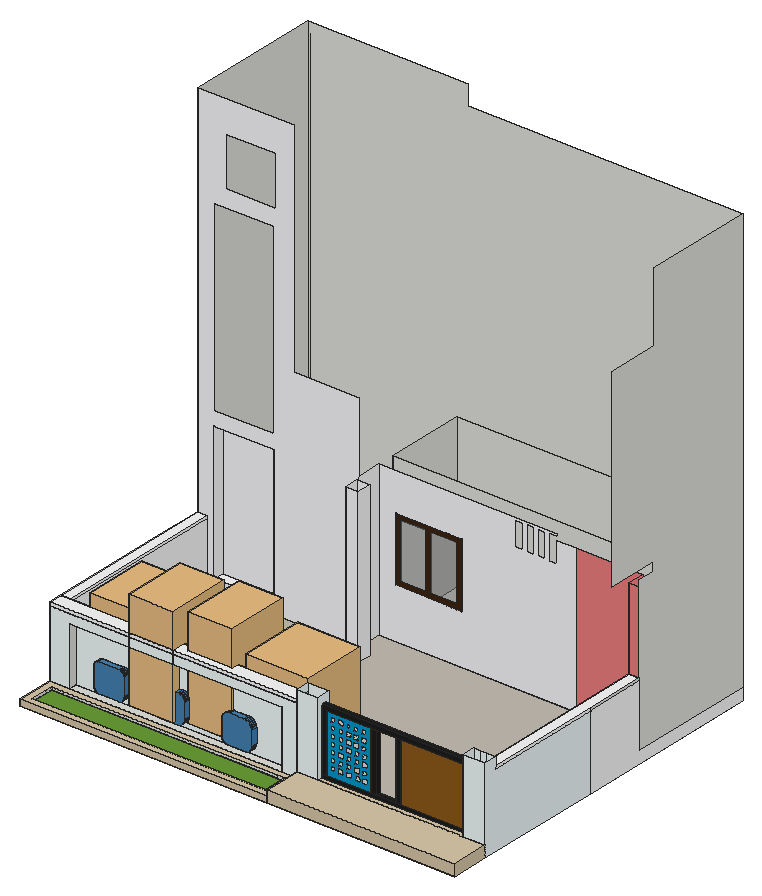
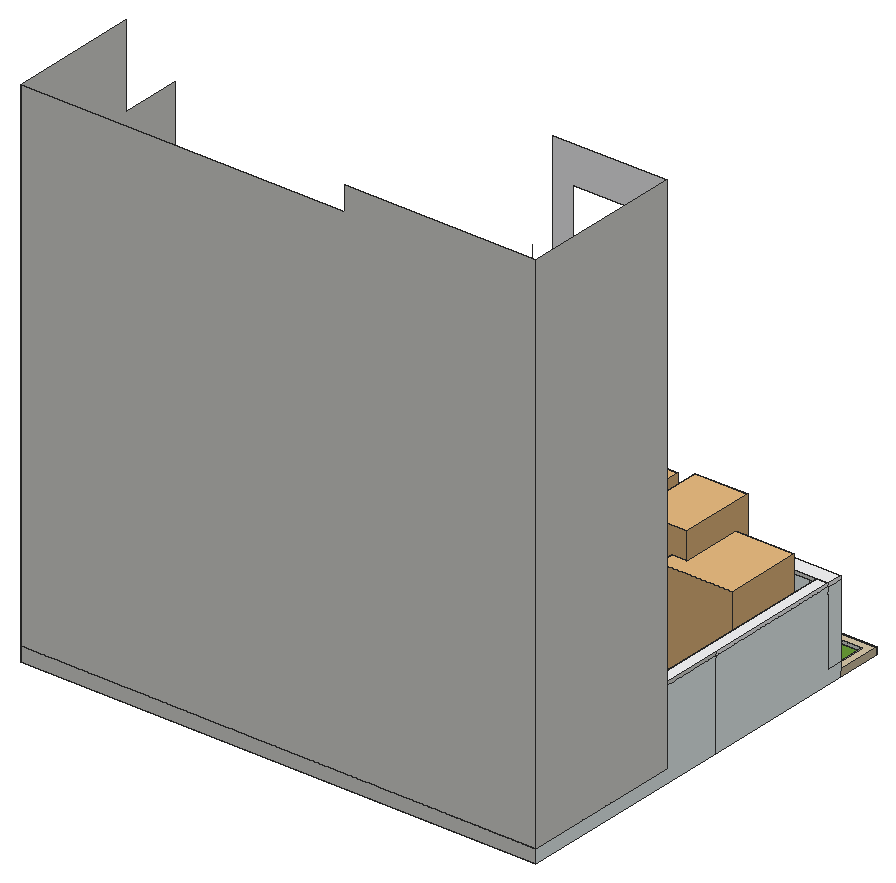
# SketchUp Ruby script. Lengths in inches.
U = 1.inch
M = Sketchup.active_model
def pt(a) = Geom::Point3d.new(a.map { |v| v * U })
def face(e, loops, mat)
  f = e.add_face(loops[0].map { |a| pt(a) })
  loops[1..].each { |l| e.add_face(l.map { |a| pt(a) }).erase! }
  f.material = f.back_material = mat if mat
  f
end
# faces: each face lists its corners as indices into pts; further lists are holes
def faces(e, pts, list, mat = nil) = list.each { |f| face(e, (f[0].is_a?(Array) ? f : [f]).map { |l| l.map { |i| pts[i] } }, mat) }
# xy, xz, yz: faces in a plane at the given z, y or x. An outline is a flat list of corners, or four numbers for a rectangle; further outlines are holes
def ring(l) = l.size == 4 ? [[l[0], l[1]], [l[2], l[1]], [l[2], l[3]], [l[0], l[3]]] : l.each_slice(2).to_a
def flat(e, list, mat, &to3) = list.each { |f| face(e, (f[0].is_a?(Array) ? f : [f]).map { |l| ring(l).map { |u, v| to3.(u, v) } }, mat) }
def xy(e, z, list, mat = nil) = flat(e, list, mat) { |x, y| [x, y, z] }
def xz(e, y, list, mat = nil) = flat(e, list, mat) { |x, z| [x, y, z] }
def yz(e, x, list, mat = nil) = flat(e, list, mat) { |y, z| [x, y, z] }
def lines(e, pts, list) = list.each { |a, b| e.add_line(pt(pts[a]), pt(pts[b])) }
# prism: a flat outline (further loops are holes) pulled along v
def prism(e, loops, v, mat = nil)
  f = face(e, loops, mat); d = Geom::Vector3d.new(v.map { |x| x * U })
  f.pushpull(f.normal.samedirection?(d) ? d.length : -d.length)
end
def box(e, o, s, mat = nil) = prism(e, [[o, [o[0] + s[0], o[1], o[2]], [o[0] + s[0], o[1] + s[1], o[2]], [o[0], o[1] + s[1], o[2]]]], [0, 0, s[2]], mat)
def at(x, y, z, deg = 0) = Geom::Transformation.translation(pt([x, y, z])) * Geom::Transformation.rotation(ORIGIN, Z_AXIS, deg.degrees)
def axes(o, x, y, z) = Geom::Transformation.new([*x, 0, *y, 0, *z, 0, *pt(o).to_a, 1])
def part(name) = M.definitions.add(name)
# library, detail: a bought-in or finely detailed component or shape, given as its bounding box
def library(name, o, s) = part(name).tap { |d| box(d.entities, o, s) }
def detail(e, o, s) = box(e.add_group.entities, o, s)
def put(e, d, t, mat = nil) = e.add_instance(d, t).tap { |i| i.material = mat if mat }
def group(e, t, mat = nil) = e.add_group.tap { |g| g.transformation = t; g.material = mat if mat }.entities
root = M.entities
M.materials.add("[0013_LightCoral]").color = [255, 136, 136]
M.materials.add("[0013_LightCoral]1").color = [240, 128, 128]
M.materials.add("[0097_DeepSkyBlue]").color = [0, 152, 204]
M.materials.add("[0100_SteelBlue]").color = [70, 130, 180]
M.materials.add("[Blinds Vertical Pattern]").color = [250, 250, 252]
M.materials.add("[Blinds Weave]").color = [141, 91, 25]
M.materials.add("[Color M08]").color = [30, 30, 30]
M.materials.add("[Field Rectangle Tile]").color = [196, 189, 179]
M.materials.add("[Field Square Tile]").color = [217, 201, 169]
M.materials.add("[Grass Dark Green]").color = [106, 157, 55]
M.materials.add("[Translucent Glass Gray]").color = [128, 128, 128]
M.materials["[Translucent Glass Gray]"].alpha = 0.5
M.materials.add("[White Subway Tile]").color = [243, 252, 253]
M.materials.add("[Wood Cherry Original]").color = [66, 37, 18]
c1 = library("chau cay",[-24.34,-109.24,0],[56.46,62.58,79.69])
c2 = library("Flora+17",[-57.52,158.6,-38.64],[66.99,62.88,77.28])
xy(root,0,[[[5.9375,0,199.85,29.3125],[11.12,5.18,194.66,24.13]],[11.12,5.18,194.66,24.13],[5.9375,29.3125,5.9375,132.68,347.47,132.68,347.47,29.3125,187.7,29.3125,187.7,35.625,21.2,35.625,21.2,29.3125],[21.2,29.3125,187.7,35.625],[5.9375,132.68,347.47,281.71]])
xy(root,0,[[199.85,0,347.47,29.3125]],"[Field Square Tile]")
xy(root,2.5,[[11.12,5.18,194.66,24.13]],"[Grass Dark Green]")
xy(root,4.6875,[[21.2,29.3125,187.7,35.625]])
xy(root,4.6875,[[[5.9375,0,199.85,29.3125],[11.12,5.18,194.66,24.13]]],"[Field Square Tile]")
xy(root,7.5625,[[43.19,31.25,57.63,35.625],[92.19,31.25,104.38,35.625],[143.86,31.25,157.93,35.625]],"[0100_SteelBlue]")
xy(root,9,[[216.33,32.96,330.16,36.41],[216.33,36.41,330.16,39.87],[133.75,159.42,143.75,170.29],[5.9375,173.82,5.9375,281.71,347.47,281.71,347.47,180.38,339.34,180.38,339.34,194.19,308.22,194.19,308.22,207.2,339.34,207.2,339.34,270.27,17.38,270.27,17.38,173.82],[17.38,173.82,17.38,270.27,132.29,270.27,132.29,207.2,308.22,207.2,308.22,194.19,132.29,194.19,132.29,173.82],
  [132.29,207.2,339.34,270.27]])
xy(root,9,[[[13.63,39.87,339.34,39.87,339.34,194.19,132.29,194.19,132.29,173.82,13.63,173.82],[133.75,159.42,143.75,170.29]]],"[Field Rectangle Tile]")
xy(root,9,[[199.85,0,347.47,29.3125],[216.33,29.3125,330.16,32.96]],"[Field Square Tile]")
xy(root,11.5,[[216.33,32.96,219.96,36.41],[219.96,32.96,255,36.41],[255,32.96,259.13,36.41],[274.16,32.96,278.35,36.41],[278.35,32.96,326.78,36.41],
  [326.78,32.96,330.16,36.41]])
xy(root,11.5,[[259.13,32.96,274.16,36.41]],"[Color M08]")
xy(root,17.61,[[19.23,173.82,65.86,182.32]],"[Blinds Vertical Pattern]")
xy(root,30.1875,[[42.77,31.25,59.07,35.625],[91.14,31.25,105.43,35.625],[145.77,31.25,156.82,35.625]],"[0100_SteelBlue]")
xy(root,50.25,[[21.2,29.3125,187.7,35.625]])
xy(root,57.36,[[255,32.96,259.13,36.41],[274.16,32.96,278.35,36.41]])
xy(root,57.36,[[259.13,32.96,274.16,36.41]],"[Color M08]")
xy(root,57.5625,[[5.9375,29.3125,199.85,39.87]])
xy(root,58.0625,[[5.9375,39.87,13.63,173.82],[339.34,39.87,347.47,180.38]])
xy(root,60.25,[[5.9375,29.3125,199.85,39.87],[5.9375,39.87,13.63,173.82]],"[Blinds Vertical Pattern]")
xy(root,60.3125,[[339.34,39.87,347.47,180.38]],"[Blinds Vertical Pattern]")
xy(root,60.88,[[216.33,32.96,326.78,36.41],[326.78,32.96,330.16,36.41]],"[Color M08]")
xz(root,0,[[5.9375,0,199.85,4.6875],[199.85,0,347.47,9]],"[Field Square Tile]")
xz(root,5.18,[[11.12,0,194.66,2.5],[11.12,2.5,194.66,4.6875]])
xz(root,24.13,[[11.12,0,21.2,2.5],[21.2,0,187.7,2.5],[187.7,0,194.66,2.5],[11.12,2.5,21.2,4.6875],[21.2,2.5,187.7,4.6875],
  [187.7,2.5,194.66,4.6875]])
xz(root,29.3125,[[5.9375,0,21.2,4.6875],[21.2,0,187.7,4.6875],[187.7,0,199.85,4.6875],[199.85,0,216.33,9],[216.33,0,330.16,9],
  [330.16,0,347.47,9]])
xz(root,29.3125,[[5.9375,57.5625,199.85,60.25]],"[Blinds Vertical Pattern]")
xz(root,29.3125,[[5.9375,4.6875,21.2,4.6875,21.2,50.25,187.7,50.25,187.7,4.6875,199.85,4.6875,199.85,57.5625,5.9375,57.5625],[199.85,9,216.33,66.6875],[330.16,9,347.47,66.6875]],"[White Subway Tile]")
xz(root,31.25,[[43.19,7.5625,57.63,7.5625,58.31,7.61,58.97,7.74,59.61,7.96,60.21,8.25,60.77,8.63,61.28,9.07,61.72,9.58,62.1,10.14,62.4,10.75,62.61,11.39,62.75,12.05,62.79,12.72,62.79,26.47,62.76,26.96,62.66,27.43,62.51,27.89,62.29,28.33,62.02,28.73,61.7,29.1,61.34,29.42,60.93,29.69,60.5,29.91,60.04,30.0625,59.56,30.16,59.07,30.1875,42.77,30.1875,42.26,30.15,41.75,30.05,41.27,29.89,40.81,29.66,40.38,29.38,40,29.04,39.66,28.66,39.375,28.23,39.15,27.77,38.99,27.29,38.89,26.78,38.85,26.27,38.85,11.91,38.89,11.34,39,10.78,39.18,10.24,39.43,9.73,39.75,9.26,40.125,8.84,40.55,8.46,41.02,8.14,41.53,7.89,42.07,7.71,42.63,7.6],[92.19,7.5625,104.38,7.5625,105.17,7.61,105.94,7.77,106.69,8.02,107.4,8.37,108.05,8.81,108.65,9.33,109.17,9.92,109.61,10.58,109.96,11.29,110.21,12.03,110.36,12.81,110.41,13.59,110.41,25.21,110.37,25.86,110.24,26.5,110.04,27.11,109.75,27.7,109.39,28.24,108.96,28.73,108.47,29.16,107.92,29.52,107.34,29.81,106.72,30.02,106.08,30.15,105.43,30.1875,91.14,30.1875,90.53,30.15,89.93,30.03,89.36,29.83,88.81,29.5625,88.3,29.22,87.84,28.82,87.44,28.36,87.1,27.86,86.83,27.31,86.64,26.73,86.52,26.13,86.48,25.52,86.48,13.28,86.53,12.53,86.67,11.8,86.91,11.09,87.24,10.42,87.66,9.8,88.15,9.24,88.71,8.74,89.33,8.33,90.01,8,90.71,7.76,91.45,7.61],[143.86,7.5625,157.93,7.5625,158.56,7.6,159.18,7.73,159.79,7.93,160.36,8.21,160.89,8.57,161.36,8.99,161.78,9.47,162.14,10,162.42,10.57,162.625,11.17,162.75,11.79,162.79,12.43,162.79,24.22,162.74,25,162.59,25.76,162.33,26.5,161.99,27.2,161.55,27.85,161.04,28.4375,160.45,28.95,159.8,29.39,159.1,29.73,158.36,29.98,157.6,30.14,156.82,30.1875,145.77,30.1875,144.86,30.13,143.98,29.95,143.12,29.66,142.31,29.26,141.56,28.76,140.88,28.16,140.28,27.48,139.78,26.73,139.38,25.92,139.09,25.0625,138.91,24.18,138.85,23.27,138.85,12.57,138.89,11.92,139.02,11.27,139.23,10.65,139.52,10.07,139.89,9.52,140.32,9.03,140.81,8.6,141.35,8.23,141.94,7.94,142.5625,7.73,143.2,7.61]],"[0100_SteelBlue]")
xz(root,32.96,[[223.16,16.5,226.22,19.56],[229.97,16.5,233.03,19.56],[236.16,16.5,239.22,19.56],[242.84,16.5,245.91,19.56],[248.47,16.5,251.53,19.56],
  [223.16,22.19,226.22,25.25],[229.91,22.19,232.97,25.25],[236.09,22.19,239.16,25.25],[242.59,22.19,245.66,25.25],[248.47,22.19,251.53,25.25],
  [223.16,27.87,226.22,30.94],[229.72,27.87,232.78,30.94],[235.91,27.87,238.97,30.94],[242.34,27.87,245.41,30.94],[248.34,27.87,251.41,30.94],
  [223.16,33.56,226.22,36.62],[229.59,33.56,232.66,36.62],[235.84,33.56,238.91,36.62],[242.16,33.56,245.22,36.62],[248.28,33.56,251.34,36.62],
  [223.16,39.25,226.22,42.31],[229.47,39.25,232.53,42.31],[235.72,39.25,238.78,42.31],[241.78,39.25,244.84,42.31],[247.97,39.25,251.03,42.31],
  [223.16,44.94,226.22,48],[229.41,44.94,232.47,48],[235.66,44.94,238.72,48],[241.72,44.94,244.78,48],[247.84,44.94,250.91,48],
  [223.16,50.75,226.22,53.81],[229.34,50.75,232.41,53.81],[235.59,50.75,238.66,53.81],[241.59,50.75,244.66,53.81],[247.53,50.75,250.59,53.81]])
xz(root,32.96,[[[219.96,11.5,255,57.36],[223.16,50.75,226.22,53.81],[223.16,44.94,226.22,48],[223.16,39.25,226.22,42.31],[223.16,33.56,226.22,36.62],[223.16,27.87,226.22,30.94],[223.16,22.19,226.22,25.25],[223.16,16.5,226.22,19.56],[229.97,16.5,233.03,19.56],[236.16,16.5,239.22,19.56],[242.84,16.5,245.91,19.56],[248.47,16.5,251.53,19.56],[229.91,22.19,232.97,25.25],[236.09,22.19,239.16,25.25],[242.59,22.19,245.66,25.25],[248.47,22.19,251.53,25.25],[229.72,27.87,232.78,30.94],[235.91,27.87,238.97,30.94],[242.34,27.87,245.41,30.94],[248.34,27.87,251.41,30.94],[229.59,33.56,232.66,36.62],[235.84,33.56,238.91,36.62],[242.16,33.56,245.22,36.62],[248.28,33.56,251.34,36.62],[229.47,39.25,232.53,42.31],[235.72,39.25,238.78,42.31],[241.78,39.25,244.84,42.31],[247.97,39.25,251.03,42.31],[229.41,44.94,232.47,48],[235.66,44.94,238.72,48],[241.72,44.94,244.78,48],[247.84,44.94,250.91,48],[229.34,50.75,232.41,53.81],[235.59,50.75,238.66,53.81],[241.59,50.75,244.66,53.81],[247.53,50.75,250.59,53.81]]],"[0097_DeepSkyBlue]")
xz(root,32.96,[[278.35,11.5,326.78,57.36]],"[Blinds Weave]")
xz(root,32.96,[[216.33,9,330.16,11.5],[216.33,11.5,219.96,11.5,219.96,57.36,326.78,57.36,326.78,60.88,216.33,60.88],[255,11.5,259.13,57.36],[274.16,11.5,278.35,57.36],[326.78,11.5,330.16,60.88]],"[Color M08]")
xz(root,35.625,[[21.2,0,187.7,4.6875],[43.19,7.5625,42.63,7.6,42.07,7.71,41.53,7.89,41.02,8.14,40.55,8.46,40.125,8.84,39.75,9.26,39.43,9.73,39.18,10.24,39,10.78,38.89,11.34,38.85,11.91,38.85,26.27,38.89,26.78,38.99,27.29,39.15,27.77,39.375,28.23,39.66,28.66,40,29.04,40.38,29.38,40.81,29.66,41.27,29.89,41.75,30.05,42.26,30.15,42.77,30.1875,59.07,30.1875,59.56,30.16,60.04,30.0625,60.5,29.91,60.93,29.69,61.34,29.42,61.7,29.1,62.02,28.73,62.29,28.33,62.51,27.89,62.66,27.43,62.76,26.96,62.79,26.47,62.79,12.72,62.75,12.05,62.61,11.39,62.4,10.75,62.1,10.14,61.72,9.58,61.28,9.07,60.77,8.63,60.21,8.25,59.61,7.96,58.97,7.74,58.31,7.61,57.63,7.5625],[92.19,7.5625,91.45,7.61,90.71,7.76,90.01,8,89.33,8.33,88.71,8.74,88.15,9.24,87.66,9.8,87.24,10.42,86.91,11.09,86.67,11.8,86.53,12.53,86.48,13.28,86.48,25.52,86.52,26.13,86.64,26.73,86.83,27.31,87.1,27.86,87.44,28.36,87.84,28.82,88.3,29.22,88.81,29.5625,89.36,29.83,89.93,30.03,90.53,30.15,91.14,30.1875,105.43,30.1875,106.08,30.15,106.72,30.02,107.34,29.81,107.92,29.52,108.47,29.16,108.96,28.73,109.39,28.24,109.75,27.7,110.04,27.11,110.24,26.5,110.37,25.86,110.41,25.21,110.41,13.59,110.36,12.81,110.21,12.03,109.96,11.29,109.61,10.58,109.17,9.92,108.65,9.33,108.05,8.81,107.4,8.37,106.69,8.02,105.94,7.77,105.17,7.61,104.38,7.5625],[143.86,7.5625,143.2,7.61,142.5625,7.73,141.94,7.94,141.35,8.23,140.81,8.6,140.32,9.03,139.89,9.52,139.52,10.07,139.23,10.65,139.02,11.27,138.89,11.92,138.85,12.57,138.85,23.27,138.91,24.18,139.09,25.0625,139.38,25.92,139.78,26.73,140.28,27.48,140.88,28.16,141.56,28.76,142.31,29.26,143.12,29.66,143.98,29.95,144.86,30.13,145.77,30.1875,156.82,30.1875,157.6,30.14,158.36,29.98,159.1,29.73,159.8,29.39,160.45,28.95,161.04,28.4375,161.55,27.85,161.99,27.2,162.33,26.5,162.59,25.76,162.74,25,162.79,24.22,162.79,12.43,162.75,11.79,162.625,11.17,162.42,10.57,162.14,10,161.78,9.47,161.36,8.99,160.89,8.57,160.36,8.21,159.79,7.93,159.18,7.73,158.56,7.6,157.93,7.5625]])
xz(root,35.625,[[[21.2,4.6875,187.7,50.25],[43.19,7.5625,42.63,7.6,42.07,7.71,41.53,7.89,41.02,8.14,40.55,8.46,40.125,8.84,39.75,9.26,39.43,9.73,39.18,10.24,39,10.78,38.89,11.34,38.85,11.91,38.85,26.27,38.89,26.78,38.99,27.29,39.15,27.77,39.375,28.23,39.66,28.66,40,29.04,40.38,29.38,40.81,29.66,41.27,29.89,41.75,30.05,42.26,30.15,42.77,30.1875,59.07,30.1875,59.56,30.16,60.04,30.0625,60.5,29.91,60.93,29.69,61.34,29.42,61.7,29.1,62.02,28.73,62.29,28.33,62.51,27.89,62.66,27.43,62.76,26.96,62.79,26.47,62.79,12.72,62.75,12.05,62.61,11.39,62.4,10.75,62.1,10.14,61.72,9.58,61.28,9.07,60.77,8.63,60.21,8.25,59.61,7.96,58.97,7.74,58.31,7.61,57.63,7.5625],[92.19,7.5625,91.45,7.61,90.71,7.76,90.01,8,89.33,8.33,88.71,8.74,88.15,9.24,87.66,9.8,87.24,10.42,86.91,11.09,86.67,11.8,86.53,12.53,86.48,13.28,86.48,25.52,86.52,26.13,86.64,26.73,86.83,27.31,87.1,27.86,87.44,28.36,87.84,28.82,88.3,29.22,88.81,29.5625,89.36,29.83,89.93,30.03,90.53,30.15,91.14,30.1875,105.43,30.1875,106.08,30.15,106.72,30.02,107.34,29.81,107.92,29.52,108.47,29.16,108.96,28.73,109.39,28.24,109.75,27.7,110.04,27.11,110.24,26.5,110.37,25.86,110.41,25.21,110.41,13.59,110.36,12.81,110.21,12.03,109.96,11.29,109.61,10.58,109.17,9.92,108.65,9.33,108.05,8.81,107.4,8.37,106.69,8.02,105.94,7.77,105.17,7.61,104.38,7.5625],[143.86,7.5625,143.2,7.61,142.5625,7.73,141.94,7.94,141.35,8.23,140.81,8.6,140.32,9.03,139.89,9.52,139.52,10.07,139.23,10.65,139.02,11.27,138.89,11.92,138.85,12.57,138.85,23.27,138.91,24.18,139.09,25.0625,139.38,25.92,139.78,26.73,140.28,27.48,140.88,28.16,141.56,28.76,142.31,29.26,143.12,29.66,143.98,29.95,144.86,30.13,145.77,30.1875,156.82,30.1875,157.6,30.14,158.36,29.98,159.1,29.73,159.8,29.39,160.45,28.95,161.04,28.4375,161.55,27.85,161.99,27.2,162.33,26.5,162.59,25.76,162.74,25,162.79,24.22,162.79,12.43,162.75,11.79,162.625,11.17,162.42,10.57,162.14,10,161.78,9.47,161.36,8.99,160.89,8.57,160.36,8.21,159.79,7.93,159.18,7.73,158.56,7.6,157.93,7.5625]]],"[White Subway Tile]")
xz(root,36.41,[[219.96,11.5,255,57.36]])
xz(root,36.41,[[278.35,11.5,326.78,57.36]],"[Blinds Weave]")
xz(root,36.41,[[216.33,9,330.16,11.5],[216.33,11.5,216.33,60.88,326.78,60.88,326.78,57.36,219.96,57.36,219.96,11.5],[255,11.5,259.13,57.36],[274.16,11.5,278.35,57.36],[326.78,11.5,330.16,60.88]],"[Color M08]")
xz(root,39.87,[[5.9375,9,13.63,57.5625],[5.9375,57.5625,13.63,58.0625],[13.63,57.5625,199.85,60.25],[5.9375,58.0625,13.63,60.25],[339.34,58.0625,347.47,60.3125]])
xz(root,39.87,[[13.63,9,199.85,57.5625],[199.85,9,216.33,66.6875],[330.16,9,334.94,66.6875],[334.94,9,339.34,66.6875],[339.34,60.3125,347.47,66.6875]],"[White Subway Tile]")
xz(root,159.42,[[133.75,9,143.75,129]],"[Blinds Vertical Pattern]")
xz(root,170.29,[[133.75,9,143.75,129]],"[Blinds Vertical Pattern]")
xz(root,173.82,[[5.9375,9,13.63,58.0625],[5.9375,58.0625,13.63,60.25]])
xz(root,173.82,[[[13.63,9,132.29,9,132.29,184.75,81.27,184.84,81.27,358.25,5.9375,358.25,5.9375,60.25,13.63,60.25],[18.61,135.61,65.8,281.86],[19.23,17.61,65.86,125.11],[28.5625,294.76,67.5625,333.76]]],"[Blinds Vertical Pattern]")
xz(root,180.38,[[339.34,9,347.47,58.0625],[339.34,58.0625,347.47,60.3125]])
xz(root,180.38,[[339.34,60.3125,347.47,124.1875]],"[0013_LightCoral]1")
xz(root,182.32,[[19.23,17.61,65.86,125.11]],"[Blinds Vertical Pattern]")
xz(root,194.19,[[287,9,339.34,124.1875]],"[0013_LightCoral]1")
xz(root,194.19,[[[132.29,9,287,9,287,124.1875,271.55,124.1875,271.55,108.13,265.86,108.13,265.86,127.39,271.54,127.39,271.54,129,132.29,129],[145.06,48.27,197.47,99.57],[256.61,108.13,262.3,127.39],[247.86,108.13,253.55,127.39],[239.11,108.13,244.8,127.39]]],"[Blinds Vertical Pattern]")
xz(root,194.19,[[149.26,51.9,168.59,95.95],[173.12,51.9,193.28,95.95]],"[Translucent Glass Gray]")
xz(root,194.19,[[[145.06,48.27,197.47,99.57],[149.26,51.9,193.28,95.95]],[168.59,51.9,173.12,95.95]],"[Wood Cherry Original]")
xz(root,207.2,[[[132.29,9,339.34,129],[158.57,39.15,218.13,106.65]]])
xz(root,270.27,[[132.29,9,339.34,129]])
xz(root,281.71,[[5.9375,0,347.47,9],[5.9375,9,5.9375,358.25,132.29,358.25,132.29,342.375,347.47,342.375,347.47,9]])
yz(root,5.9375,[[173.82,9,281.71,358.25],[132.68,58.0625,173.82,60.25]])
yz(root,5.9375,[[29.3125,57.5625,39.87,60.25],[39.87,58.0625,132.68,60.25]],"[Blinds Vertical Pattern]")
yz(root,5.9375,[[0,0,29.3125,4.6875]],"[Field Square Tile]")
yz(root,5.9375,[[29.3125,0,29.3125,9,39.87,9,39.87,58.0625,132.68,58.0625,132.68,0],[132.68,0,132.68,58.0625,173.82,58.0625,173.82,9,281.71,9,281.71,0],[29.3125,9,39.87,57.5625]],"[White Subway Tile]")
yz(root,11.12,[[5.18,0,24.13,2.5],[5.18,2.5,24.13,4.6875]])
yz(root,13.63,[[39.87,9,173.82,58.0625],[39.87,58.0625,173.82,60.25]],"[Blinds Vertical Pattern]")
yz(root,19.23,[[173.82,17.61,182.32,125.11]],"[Blinds Vertical Pattern]")
yz(root,21.2,[[29.3125,0,35.625,4.6875],[29.3125,4.6875,35.625,50.25]])
yz(root,38.85,[[31.25,11.91,35.625,26.27]],"[0100_SteelBlue]")
yz(root,62.79,[[31.25,12.72,35.625,26.47]],"[0100_SteelBlue]")
yz(root,65.86,[[173.82,17.61,182.32,125.11]],"[Blinds Vertical Pattern]")
yz(root,86.48,[[31.25,13.28,35.625,25.52]],"[0100_SteelBlue]")
yz(root,110.41,[[31.25,13.59,35.625,25.21]],"[0100_SteelBlue]")
yz(root,132.29,[[207.2,9,270.27,129]])
yz(root,132.29,[[173.82,9,194.19,129]],"[Blinds Vertical Pattern]")
yz(root,133.75,[[159.42,9,170.29,129]],"[Blinds Vertical Pattern]")
yz(root,138.85,[[31.25,12.57,35.625,23.27]],"[0100_SteelBlue]")
yz(root,143.75,[[159.42,9,170.29,129]],"[Blinds Vertical Pattern]")
yz(root,162.79,[[31.25,12.43,35.625,24.22]],"[0100_SteelBlue]")
yz(root,187.7,[[29.3125,0,35.625,4.6875],[29.3125,4.6875,35.625,50.25]])
yz(root,194.66,[[5.18,0,24.13,2.5],[5.18,2.5,24.13,4.6875]])
yz(root,199.85,[[0,0,29.3125,4.6875],[29.3125,9,39.87,57.5625],[29.3125,57.5625,39.87,60.25]])
yz(root,199.85,[[0,4.6875,29.3125,9]],"[Field Square Tile]")
yz(root,199.85,[[29.3125,60.25,39.87,66.6875]],"[White Subway Tile]")
yz(root,216.33,[[32.96,9,36.41,11.5],[32.96,11.5,36.41,60.88]])
yz(root,216.33,[[29.3125,9,32.96,9,32.96,60.88,36.41,60.88,36.41,9,39.87,9,39.87,66.6875,29.3125,66.6875]],"[White Subway Tile]")
yz(root,219.96,[[32.96,11.5,36.41,57.36]])
yz(root,255,[[32.96,11.5,36.41,57.36]])
yz(root,259.13,[[32.96,11.5,36.41,57.36]],"[Color M08]")
yz(root,274.16,[[32.96,11.5,36.41,57.36]],"[Color M08]")
yz(root,278.35,[[32.96,11.5,36.41,57.36]])
yz(root,326.78,[[32.96,11.5,36.41,57.36]])
yz(root,330.16,[[32.96,9,36.41,11.5],[32.96,11.5,36.41,60.88]])
yz(root,330.16,[[29.3125,9,29.3125,66.6875,39.87,66.6875,39.87,9,36.41,9,36.41,60.88,32.96,60.88,32.96,9]],"[White Subway Tile]")
yz(root,339.34,[[207.2,9,270.27,129]])
yz(root,339.34,[[180.38,9,194.19,124.1875]],"[0013_LightCoral]")
yz(root,339.34,[[39.87,9,180.38,58.0625],[39.87,58.0625,180.38,60.3125]],"[Blinds Vertical Pattern]")
yz(root,347.47,[[180.38,9,281.71,9,281.71,342.375,194.64,342.375,194.64,287.6875,153.45,287.6875,153.45,136,194.19,136,194.19,129,180.38,129],[132.68,58.0625,180.38,60.3125]])
yz(root,347.47,[[132.68,0,281.71,0,281.71,9,180.38,9,180.38,58.0625,132.68,58.0625],[39.87,58.0625,132.68,60.3125]],"[Blinds Vertical Pattern]")
yz(root,347.47,[[0,0,29.3125,9]],"[Field Square Tile]")
yz(root,347.47,[[29.3125,0,132.68,0,132.68,58.0625,39.87,58.0625,39.87,66.6875,29.3125,66.6875]],"[White Subway Tile]")
p = [[42.07,35.625,7.71],[42.63,35.625,7.6],[42.63,31.25,7.6],[42.07,31.25,7.71],[43.19,35.625,7.5625],[43.19,31.25,7.5625],
  [57.63,35.625,7.5625],[58.31,35.625,7.61],[58.31,31.25,7.61],[57.63,31.25,7.5625],[58.97,35.625,7.74],[58.97,31.25,7.74],
  [90.71,35.625,7.76],[91.45,35.625,7.61],[91.45,31.25,7.61],[90.71,31.25,7.76],[92.19,35.625,7.5625],[92.19,31.25,7.5625],
  [104.38,35.625,7.5625],[105.17,35.625,7.61],[105.17,31.25,7.61],[104.38,31.25,7.5625],[105.94,35.625,7.77],[105.94,31.25,7.77],
  [142.5625,35.625,7.73],[143.2,35.625,7.61],[143.2,31.25,7.61],[142.5625,31.25,7.73],[143.86,35.625,7.5625],[143.86,31.25,7.5625],
  [157.93,35.625,7.5625],[158.56,35.625,7.6],[158.56,31.25,7.6],[157.93,31.25,7.5625],[159.18,35.625,7.73],[159.18,31.25,7.73],
  [41.53,35.625,7.89],[41.53,31.25,7.89],[59.61,35.625,7.96],[59.61,31.25,7.96],[141.94,35.625,7.94],[141.94,31.25,7.94],
  [159.79,35.625,7.93],[159.79,31.25,7.93],[90.01,35.625,8],[90.01,31.25,8],[106.69,35.625,8.02],[106.69,31.25,8.02],
  [41.02,35.625,8.14],[41.02,31.25,8.14],[141.35,35.625,8.23],[141.35,31.25,8.23],[160.36,35.625,8.21],[160.36,31.25,8.21],
  [60.21,35.625,8.25],[60.21,31.25,8.25],[89.33,35.625,8.33],[89.33,31.25,8.33],[107.4,35.625,8.37],[107.4,31.25,8.37],
  [40.55,35.625,8.46],[40.55,31.25,8.46],[140.81,35.625,8.6],[140.81,31.25,8.6],[160.89,35.625,8.57],[160.89,31.25,8.57],
  [60.77,35.625,8.63],[60.77,31.25,8.63],[88.71,35.625,8.74],[88.71,31.25,8.74],[108.05,35.625,8.81],[108.05,31.25,8.81],
  [40.125,35.625,8.84],[40.125,31.25,8.84],[61.28,35.625,9.07],[61.28,31.25,9.07],[140.32,35.625,9.03],[140.32,31.25,9.03],
  [161.36,35.625,8.99],[161.36,31.25,8.99],[88.15,35.625,9.24],[88.15,31.25,9.24],[39.75,35.625,9.26],[39.75,31.25,9.26],
  [108.65,35.625,9.33],[108.65,31.25,9.33],[139.89,35.625,9.52],[139.89,31.25,9.52],[161.78,35.625,9.47],[161.78,31.25,9.47],
  [61.72,35.625,9.58],[61.72,31.25,9.58],[87.66,35.625,9.8],[87.66,31.25,9.8],[39.43,35.625,9.73],[39.43,31.25,9.73],
  [109.17,35.625,9.92],[109.17,31.25,9.92],[139.52,35.625,10.07],[139.52,31.25,10.07],[162.14,35.625,10],[162.14,31.25,10],
  [62.1,35.625,10.14],[62.1,31.25,10.14],[39.18,35.625,10.24],[39.18,31.25,10.24],[87.24,35.625,10.42],[87.24,31.25,10.42],
  [109.61,35.625,10.58],[109.61,31.25,10.58],[162.42,35.625,10.57],[162.42,31.25,10.57],[62.4,35.625,10.75],[62.4,31.25,10.75],
  [139.23,35.625,10.65],[139.23,31.25,10.65],[39,35.625,10.78],[39,31.25,10.78],[86.91,35.625,11.09],[86.91,31.25,11.09],
  [109.96,35.625,11.29],[109.96,31.25,11.29],[162.625,35.625,11.17],[162.625,31.25,11.17],[62.61,35.625,11.39],[62.61,31.25,11.39],
  [139.02,35.625,11.27],[139.02,31.25,11.27],[38.89,35.625,11.34],[38.89,31.25,11.34],[86.67,35.625,11.8],[86.67,31.25,11.8],
  [162.75,35.625,11.79],[162.75,31.25,11.79],[38.85,35.625,11.91],[38.85,31.25,11.91],[110.21,35.625,12.03],[110.21,31.25,12.03],
  [138.89,35.625,11.92],[138.89,31.25,11.92],[62.75,35.625,12.05],[62.75,31.25,12.05],[86.53,35.625,12.53],[86.53,31.25,12.53],
  [162.79,35.625,12.43],[162.79,31.25,12.43],[138.85,35.625,12.57],[138.85,31.25,12.57],[62.79,35.625,12.72],[62.79,31.25,12.72],
  [110.36,35.625,12.81],[110.36,31.25,12.81],[86.48,35.625,13.28],[86.48,31.25,13.28],[110.41,35.625,13.59],[110.41,31.25,13.59],
  [138.91,35.625,24.18],[138.85,35.625,23.27],[138.85,31.25,23.27],[138.91,31.25,24.18],[139.09,35.625,25.0625],[139.09,31.25,25.0625],
  [162.79,35.625,24.22],[162.74,35.625,25],[162.74,31.25,25],[162.79,31.25,24.22],[162.59,35.625,25.76],[162.59,31.25,25.76],
  [139.38,35.625,25.92],[139.38,31.25,25.92],[110.41,35.625,25.21],[110.37,35.625,25.86],[110.37,31.25,25.86],[110.41,31.25,25.21],
  [86.52,35.625,26.13],[86.48,35.625,25.52],[86.48,31.25,25.52],[86.52,31.25,26.13],[162.33,35.625,26.5],[162.33,31.25,26.5],
  [110.24,35.625,26.5],[110.24,31.25,26.5],[139.78,35.625,26.73],[139.78,31.25,26.73],[86.64,35.625,26.73],[86.64,31.25,26.73],
  [38.89,35.625,26.78],[38.85,35.625,26.27],[38.85,31.25,26.27],[38.89,31.25,26.78],[62.79,35.625,26.47],[62.76,35.625,26.96],
  [62.76,31.25,26.96],[62.79,31.25,26.47],[110.04,35.625,27.11],[110.04,31.25,27.11],[161.99,35.625,27.2],[161.99,31.25,27.2],
  [86.83,35.625,27.31],[86.83,31.25,27.31],[140.28,35.625,27.48],[140.28,31.25,27.48],[38.99,35.625,27.29],[38.99,31.25,27.29],
  [62.66,35.625,27.43],[62.66,31.25,27.43],[109.75,35.625,27.7],[109.75,31.25,27.7],[161.55,35.625,27.85],[161.55,31.25,27.85],
  [39.15,35.625,27.77],[39.15,31.25,27.77],[87.1,35.625,27.86],[87.1,31.25,27.86],[62.51,35.625,27.89],[62.51,31.25,27.89],
  [140.88,35.625,28.16],[140.88,31.25,28.16],[109.39,35.625,28.24],[109.39,31.25,28.24],[39.375,35.625,28.23],[39.375,31.25,28.23],
  [62.29,35.625,28.33],[62.29,31.25,28.33],[87.44,35.625,28.36],[87.44,31.25,28.36],[161.04,35.625,28.4375],[161.04,31.25,28.4375],
  [39.66,35.625,28.66],[39.66,31.25,28.66],[108.96,35.625,28.73],[108.96,31.25,28.73],[141.56,35.625,28.76],[141.56,31.25,28.76],
  [62.02,35.625,28.73],[62.02,31.25,28.73],[87.84,35.625,28.82],[87.84,31.25,28.82],[160.45,35.625,28.95],[160.45,31.25,28.95],
  [40,35.625,29.04],[40,31.25,29.04],[61.7,35.625,29.1],[61.7,31.25,29.1],[108.47,35.625,29.16],[108.47,31.25,29.16],
  [88.3,35.625,29.22],[88.3,31.25,29.22],[142.31,35.625,29.26],[142.31,31.25,29.26],[40.38,35.625,29.38],[40.38,31.25,29.38],
  [159.8,35.625,29.39],[159.8,31.25,29.39],[61.34,35.625,29.42],[61.34,31.25,29.42],[88.81,35.625,29.5625],[88.81,31.25,29.5625],
  [107.92,35.625,29.52],[107.92,31.25,29.52],[143.12,35.625,29.66],[143.12,31.25,29.66],[40.81,35.625,29.66],[40.81,31.25,29.66],
  [60.93,35.625,29.69],[60.93,31.25,29.69],[159.1,35.625,29.73],[159.1,31.25,29.73],[107.34,35.625,29.81],[107.34,31.25,29.81],
  [89.36,35.625,29.83],[89.36,31.25,29.83],[41.27,35.625,29.89],[41.27,31.25,29.89],[60.5,35.625,29.91],[60.5,31.25,29.91],
  [143.98,35.625,29.95],[143.98,31.25,29.95],[158.36,35.625,29.98],[158.36,31.25,29.98],[89.93,35.625,30.03],[89.93,31.25,30.03],
  [106.72,35.625,30.02],[106.72,31.25,30.02],[41.75,35.625,30.05],[41.75,31.25,30.05],[60.04,35.625,30.0625],[60.04,31.25,30.0625],
  [90.53,35.625,30.15],[90.53,31.25,30.15],[106.08,35.625,30.15],[106.08,31.25,30.15],[144.86,35.625,30.13],[144.86,31.25,30.13],
  [157.6,35.625,30.14],[157.6,31.25,30.14],[42.26,35.625,30.15],[42.26,31.25,30.15],[59.56,35.625,30.16],[59.56,31.25,30.16],
  [91.14,35.625,30.1875],[91.14,31.25,30.1875],[105.43,35.625,30.1875],[105.43,31.25,30.1875],[145.77,35.625,30.1875],[145.77,31.25,30.1875],
  [156.82,35.625,30.1875],[156.82,31.25,30.1875],[42.77,35.625,30.1875],[42.77,31.25,30.1875],[59.07,35.625,30.1875],[59.07,31.25,30.1875],
  [145.06,194.19,48.27],[158.57,207.2,39.15],[158.57,207.2,106.65],[145.06,194.19,99.57],[197.47,194.19,48.27],[218.13,207.2,39.15],
  [197.47,194.19,99.57],[218.13,207.2,106.65],[17.38,270.27,9],[17.38,270.27,358.25]]
faces(root,p,[[0,1,2,3],[1,4,5,2],[6,7,8,9],[7,10,11,8],[12,13,14,15],[13,16,17,14],[18,19,20,21],[19,22,23,20],
  [24,25,26,27],[25,28,29,26],[30,31,32,33],[31,34,35,32],[36,0,3,37],[10,38,39,11],[40,24,27,41],[34,42,43,35],
  [44,12,15,45],[22,46,47,23],[48,36,37,49],[50,40,41,51],[42,52,53,43],[38,54,55,39],[56,44,45,57],[46,58,59,47],
  [60,48,49,61],[62,50,51,63],[52,64,65,53],[54,66,67,55],[68,56,57,69],[58,70,71,59],[72,60,61,73],[66,74,75,67],
  [76,62,63,77],[64,78,79,65],[80,68,69,81],[82,72,73,83],[70,84,85,71],[86,76,77,87],[78,88,89,79],[74,90,91,75],
  [92,80,81,93],[94,82,83,95],[84,96,97,85],[98,86,87,99],[88,100,101,89],[90,102,103,91],[104,94,95,105],[106,92,93,107],
  [96,108,109,97],[100,110,111,101],[102,112,113,103],[114,98,99,115],[116,104,105,117],[118,106,107,119],[108,120,121,109],[110,122,123,111],
  [112,124,125,113],[126,114,115,127],[128,116,117,129],[130,118,119,131],[122,132,133,123],[134,128,129,135],[120,136,137,121],[138,126,127,139],
  [124,140,141,125],[142,130,131,143],[132,144,145,133],[146,138,139,147],[140,148,149,141],[136,150,151,137],[152,142,143,153],[150,154,155,151],
  [156,157,158,159],[160,156,159,161],[162,163,164,165],[163,166,167,164],[168,160,161,169],[170,171,172,173],[174,175,176,177],[166,178,179,167],
  [171,180,181,172],[182,168,169,183],[184,174,177,185],[186,187,188,189],[190,191,192,193],[180,194,195,181],[178,196,197,179],[198,184,185,199],
  [200,182,183,201],[202,186,189,203],[191,204,205,192],[194,206,207,195],[196,208,209,197],[210,202,203,211],[212,198,199,213],[204,214,215,205],
  [216,200,201,217],[206,218,219,207],[220,210,211,221],[214,222,223,215],[224,212,213,225],[208,226,227,209],[228,220,221,229],[218,230,231,219],
  [232,216,217,233],[222,234,235,223],[236,224,225,237],[226,238,239,227],[240,228,229,241],[234,242,243,235],[230,244,245,231],[246,236,237,247],
  [248,232,233,249],[250,240,241,251],[238,252,253,239],[242,254,255,243],[256,246,247,257],[244,258,259,245],[260,248,249,261],[262,250,251,263],
  [254,264,265,255],[252,266,267,253],[258,268,269,259],[270,256,257,271],[272,262,263,273],[264,274,275,265],[276,260,261,277],[266,278,279,267],
  [280,270,271,281],[268,282,283,269],[284,272,273,285],[274,286,287,275],[288,280,281,289],[282,290,291,283],[292,276,277,293],[278,294,295,279],
  [296,284,285,297],[286,298,299,287],[300,288,289,301],[290,302,303,291],[304,292,293,305],[294,306,307,295],[308,296,297,309],[298,310,311,299]],"[0100_SteelBlue]")
faces(root,p,[[312,313,314,315],[312,316,317,313],[316,318,319,317]])
lines(root,p,[[320,321]])
put(root,c1,axes([82.5,117.14,9],[0.6162,0,0],[0,0.8,0],[0,0,0.98]))
put(root,c1,axes([124.6875,122.26,9],[0.6162,0,0],[0,0.8,0],[0,0,0.98]))
put(root,c2,axes([70.49,-88.6,39.38],[0.73,0,0],[0,0.81,0],[0,0,0.78624]))
put(root,c2,axes([192.93,-88.6,39.38],[0.73,0,0],[0,0.81,0],[0,0,0.78624]))
